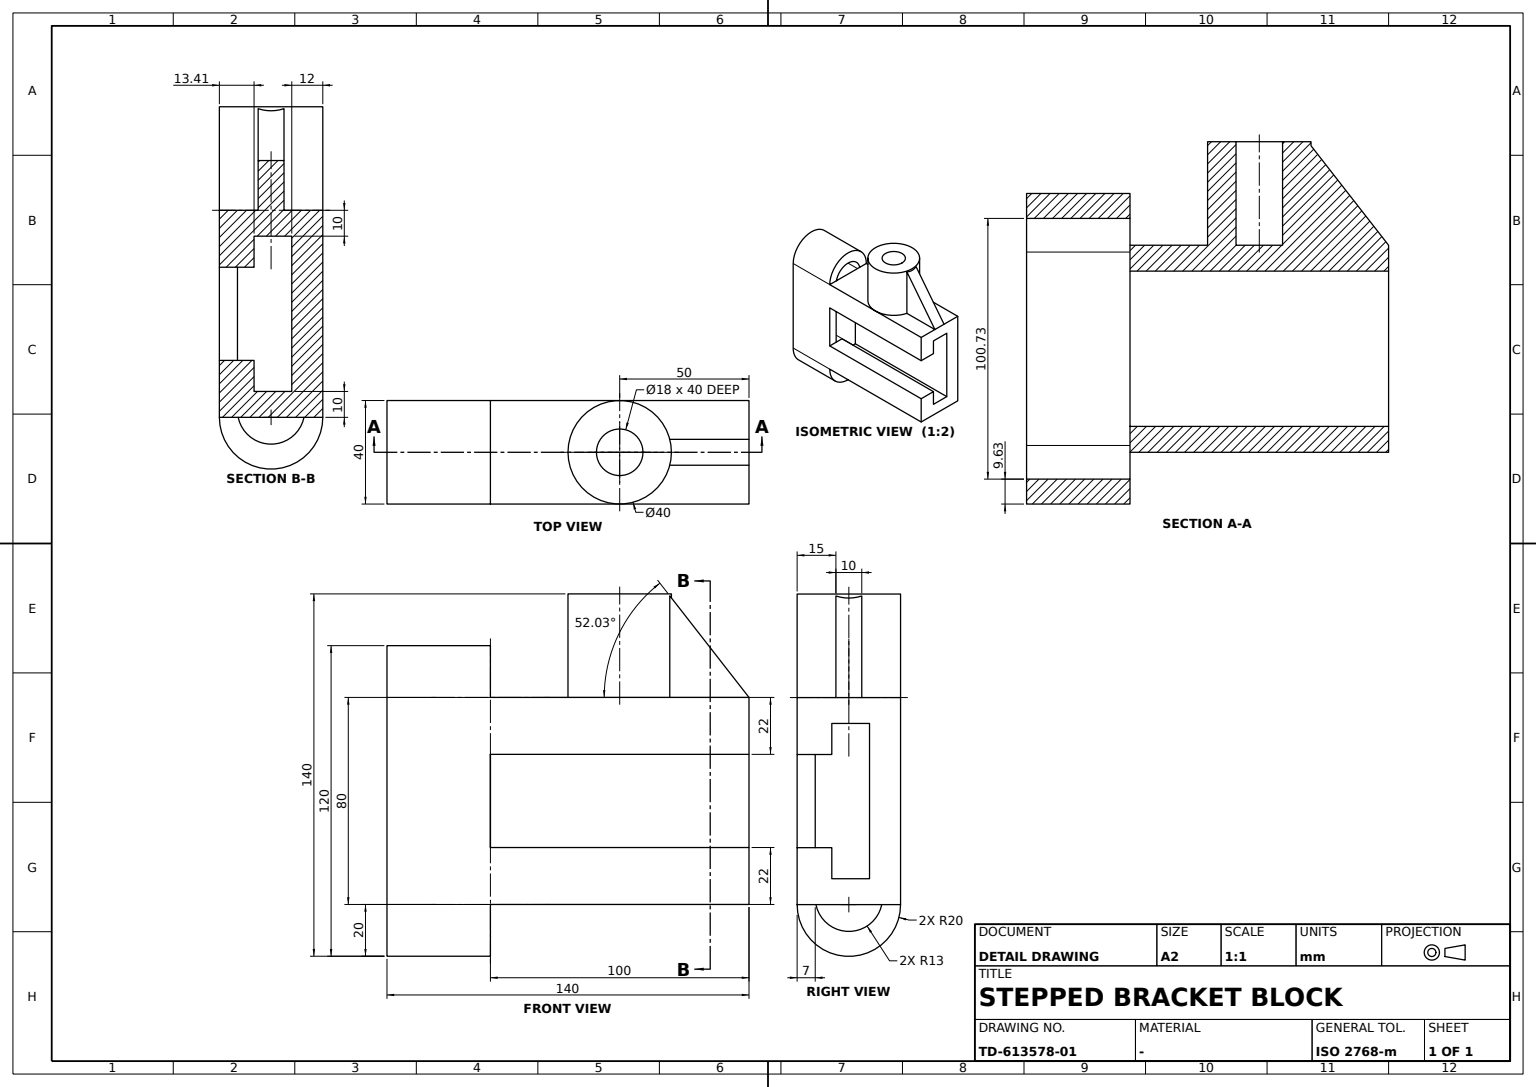
ISO-10303-21;
HEADER;
FILE_DESCRIPTION((''),'2;1');
FILE_NAME('','',(''),(''),'','','');
FILE_SCHEMA(('AUTOMOTIVE_DESIGN'));
ENDSEC;
DATA;
#1=APPLICATION_CONTEXT('');
#2=PRODUCT_CONTEXT('',#1,'mechanical');
#3=PRODUCT('','','',(#2));
#4=PRODUCT_DEFINITION_FORMATION('','',#3);
#5=PRODUCT_DEFINITION_CONTEXT('',#1,'design');
#6=PRODUCT_DEFINITION('','',#4,#5);
#7=PRODUCT_DEFINITION_SHAPE('','',#6);
#8=(LENGTH_UNIT()NAMED_UNIT(*)SI_UNIT(.MILLI.,.METRE.));
#9=(NAMED_UNIT(*)PLANE_ANGLE_UNIT()SI_UNIT($,.RADIAN.));
#10=(NAMED_UNIT(*)SI_UNIT($,.STERADIAN.)SOLID_ANGLE_UNIT());
#11=UNCERTAINTY_MEASURE_WITH_UNIT(LENGTH_MEASURE(0.005),#8,'distance_accuracy_value','');
#12=(GEOMETRIC_REPRESENTATION_CONTEXT(3)GLOBAL_UNCERTAINTY_ASSIGNED_CONTEXT((#11))GLOBAL_UNIT_ASSIGNED_CONTEXT((#8,#9,#10))REPRESENTATION_CONTEXT('',''));
#13=CARTESIAN_POINT('',(-41.,0.,40.));
#14=VERTEX_POINT('',#13);
#15=CARTESIAN_POINT('',(-50.,0.,40.));
#16=DIRECTION('',(0.,0.,1.));
#17=DIRECTION('',(1.,0.,0.));
#18=AXIS2_PLACEMENT_3D('',#15,#16,#17);
#19=CIRCLE('',#18,9.);
#20=EDGE_CURVE('',#14,#14,#19,.T.);
#21=ORIENTED_EDGE('',*,*,#20,.F.);
#22=EDGE_LOOP('',(#21));
#23=FACE_BOUND('',#22,.T.);
#24=CARTESIAN_POINT('',(-41.,0.,80.));
#25=VERTEX_POINT('',#24);
#26=CARTESIAN_POINT('',(-50.,0.,80.));
#27=AXIS2_PLACEMENT_3D('',#26,#16,#17);
#28=CIRCLE('',#27,9.);
#29=EDGE_CURVE('',#25,#25,#28,.T.);
#30=ORIENTED_EDGE('',*,*,#29,.T.);
#31=EDGE_LOOP('',(#30));
#32=FACE_BOUND('',#31,.T.);
#33=CARTESIAN_POINT('',(-50.,0.,60.));
#34=AXIS2_PLACEMENT_3D('',#33,#16,#17);
#35=CYLINDRICAL_SURFACE('',#34,9.);
#36=ADVANCED_FACE('',(#23,#32),#35,.F.);
#37=CARTESIAN_POINT('',(-100.,12.730269,40.));
#38=VERTEX_POINT('',#37);
#39=CARTESIAN_POINT('',(-100.,20.,40.));
#40=VERTEX_POINT('',#39);
#41=CARTESIAN_POINT('',(-100.,-20.,40.));
#42=DIRECTION('',(0.,1.,0.));
#43=VECTOR('',#42,1000.);
#44=LINE('',#41,#43);
#45=EDGE_CURVE('',#38,#40,#44,.T.);
#46=ORIENTED_EDGE('',*,*,#45,.T.);
#47=VERTEX_POINT('',#41);
#48=CARTESIAN_POINT('',(-100.,0.,40.));
#49=DIRECTION('',(0.,0.,-1.));
#50=AXIS2_PLACEMENT_3D('',#48,#17,#49);
#51=CIRCLE('',#50,20.);
#52=EDGE_CURVE('',#40,#47,#51,.T.);
#53=ORIENTED_EDGE('',*,*,#52,.T.);
#54=CARTESIAN_POINT('',(-100.,-12.730269,40.));
#55=VERTEX_POINT('',#54);
#56=EDGE_CURVE('',#47,#55,#44,.T.);
#57=ORIENTED_EDGE('',*,*,#56,.T.);
#58=CARTESIAN_POINT('',(-100.,0.,37.365564));
#59=AXIS2_PLACEMENT_3D('',#58,#17,#49);
#60=CIRCLE('',#59,13.);
#61=EDGE_CURVE('',#55,#38,#60,.F.);
#62=ORIENTED_EDGE('',*,*,#61,.T.);
#63=EDGE_LOOP('',(#46,#53,#57,#62));
#64=FACE_BOUND('',#63,.T.);
#65=CARTESIAN_POINT('',(-100.,0.,0.));
#66=AXIS2_PLACEMENT_3D('',#65,#17,#42);
#67=PLANE('',#66);
#68=ADVANCED_FACE('',(#64),#67,.T.);
#69=CARTESIAN_POINT('',(-100.,13.,-37.365564));
#70=VERTEX_POINT('',#69);
#71=CARTESIAN_POINT('',(-100.,12.730269,-40.));
#72=VERTEX_POINT('',#71);
#73=CARTESIAN_POINT('',(-100.,0.,-37.365564));
#74=AXIS2_PLACEMENT_3D('',#73,#17,#49);
#75=CIRCLE('',#74,13.);
#76=EDGE_CURVE('',#70,#72,#75,.F.);
#77=ORIENTED_EDGE('',*,*,#76,.F.);
#78=CARTESIAN_POINT('',(-140.,13.,-37.365564));
#79=VERTEX_POINT('',#78);
#80=CARTESIAN_POINT('',(-120.,13.,-37.365564));
#81=DIRECTION('',(-1.,0.,0.));
#82=VECTOR('',#81,1000.);
#83=LINE('',#80,#82);
#84=EDGE_CURVE('',#79,#70,#83,.F.);
#85=ORIENTED_EDGE('',*,*,#84,.F.);
#86=CARTESIAN_POINT('',(-140.,-13.,-37.365564));
#87=VERTEX_POINT('',#86);
#88=CARTESIAN_POINT('',(-140.,0.,-37.365564));
#89=AXIS2_PLACEMENT_3D('',#88,#81,#16);
#90=CIRCLE('',#89,13.);
#91=EDGE_CURVE('',#79,#87,#90,.T.);
#92=ORIENTED_EDGE('',*,*,#91,.T.);
#93=CARTESIAN_POINT('',(-100.,-13.,-37.365564));
#94=VERTEX_POINT('',#93);
#95=CARTESIAN_POINT('',(-120.,-13.,-37.365564));
#96=LINE('',#95,#82);
#97=EDGE_CURVE('',#87,#94,#96,.F.);
#98=ORIENTED_EDGE('',*,*,#97,.T.);
#99=CARTESIAN_POINT('',(-100.,-12.730269,-40.));
#100=VERTEX_POINT('',#99);
#101=EDGE_CURVE('',#100,#94,#75,.F.);
#102=ORIENTED_EDGE('',*,*,#101,.F.);
#103=EDGE_CURVE('',#72,#100,#75,.F.);
#104=ORIENTED_EDGE('',*,*,#103,.F.);
#105=EDGE_LOOP('',(#77,#85,#92,#98,#102,#104));
#106=FACE_BOUND('',#105,.T.);
#107=CARTESIAN_POINT('',(-120.,0.,-37.365564));
#108=DIRECTION('',(0.,-1.,0.));
#109=AXIS2_PLACEMENT_3D('',#107,#81,#108);
#110=CYLINDRICAL_SURFACE('',#109,13.);
#111=ADVANCED_FACE('',(#106),#110,.F.);
#112=CARTESIAN_POINT('',(-100.,-6.587677,30.));
#113=VERTEX_POINT('',#112);
#114=CARTESIAN_POINT('',(-100.,-6.587677,18.));
#115=VERTEX_POINT('',#114);
#116=VECTOR('',#49,1000.);
#117=LINE('',#112,#116);
#118=EDGE_CURVE('',#113,#115,#117,.T.);
#119=ORIENTED_EDGE('',*,*,#118,.F.);
#120=CARTESIAN_POINT('',(0.,-6.587677,30.));
#121=VERTEX_POINT('',#120);
#122=LINE('',#120,#82);
#123=EDGE_CURVE('',#121,#113,#122,.T.);
#124=ORIENTED_EDGE('',*,*,#123,.F.);
#125=CARTESIAN_POINT('',(0.,-6.587677,18.));
#126=VERTEX_POINT('',#125);
#127=LINE('',#120,#116);
#128=EDGE_CURVE('',#121,#126,#127,.T.);
#129=ORIENTED_EDGE('',*,*,#128,.T.);
#130=LINE('',#125,#82);
#131=EDGE_CURVE('',#126,#115,#130,.T.);
#132=ORIENTED_EDGE('',*,*,#131,.T.);
#133=EDGE_LOOP('',(#119,#124,#129,#132));
#134=FACE_BOUND('',#133,.T.);
#135=AXIS2_PLACEMENT_3D('',#120,#42,#49);
#136=PLANE('',#135);
#137=ADVANCED_FACE('',(#134),#136,.T.);
#138=CARTESIAN_POINT('',(-30.635083,-5.,40.));
#139=VERTEX_POINT('',#138);
#140=CARTESIAN_POINT('',(-30.635083,-5.,79.256793));
#141=VERTEX_POINT('',#140);
#142=VECTOR('',#16,1000.);
#143=LINE('',#138,#142);
#144=EDGE_CURVE('',#139,#141,#143,.T.);
#145=ORIENTED_EDGE('',*,*,#144,.T.);
#146=CARTESIAN_POINT('',(-30.635083,5.,79.256793));
#147=VERTEX_POINT('',#146);
#148=CARTESIAN_POINT('',(-50.,0.,104.071627));
#149=DIRECTION('',(0.788358294,0.,0.615216385));
#150=DIRECTION('',(-0.615216385,0.,0.788358294));
#151=AXIS2_PLACEMENT_3D('',#148,#149,#150);
#152=ELLIPSE('',#151,32.508887,20.);
#153=EDGE_CURVE('',#141,#147,#152,.T.);
#154=ORIENTED_EDGE('',*,*,#153,.T.);
#155=CARTESIAN_POINT('',(-30.635083,5.,40.));
#156=VERTEX_POINT('',#155);
#157=LINE('',#155,#142);
#158=EDGE_CURVE('',#156,#147,#157,.T.);
#159=ORIENTED_EDGE('',*,*,#158,.F.);
#160=CARTESIAN_POINT('',(-50.,20.,40.));
#161=VERTEX_POINT('',#160);
#162=CIRCLE('',#18,20.);
#163=EDGE_CURVE('',#156,#161,#162,.T.);
#164=ORIENTED_EDGE('',*,*,#163,.T.);
#165=CARTESIAN_POINT('',(-50.,-20.,40.));
#166=VERTEX_POINT('',#165);
#167=EDGE_CURVE('',#161,#166,#162,.T.);
#168=ORIENTED_EDGE('',*,*,#167,.T.);
#169=EDGE_CURVE('',#166,#139,#162,.T.);
#170=ORIENTED_EDGE('',*,*,#169,.T.);
#171=EDGE_LOOP('',(#145,#154,#159,#164,#168,#170));
#172=FACE_BOUND('',#171,.T.);
#173=CARTESIAN_POINT('',(-30.,0.,80.));
#174=VERTEX_POINT('',#173);
#175=CIRCLE('',#27,20.);
#176=EDGE_CURVE('',#174,#174,#175,.T.);
#177=ORIENTED_EDGE('',*,*,#176,.F.);
#178=EDGE_LOOP('',(#177));
#179=FACE_BOUND('',#178,.T.);
#180=CYLINDRICAL_SURFACE('',#34,20.);
#181=ADVANCED_FACE('',(#172,#179),#180,.T.);
#182=CARTESIAN_POINT('',(-140.,-13.,37.365564));
#183=VERTEX_POINT('',#182);
#184=CARTESIAN_POINT('',(-140.,13.,37.365564));
#185=VERTEX_POINT('',#184);
#186=CARTESIAN_POINT('',(-140.,0.,37.365564));
#187=AXIS2_PLACEMENT_3D('',#186,#81,#16);
#188=CIRCLE('',#187,13.);
#189=EDGE_CURVE('',#183,#185,#188,.T.);
#190=ORIENTED_EDGE('',*,*,#189,.T.);
#191=CARTESIAN_POINT('',(-100.,13.,37.365564));
#192=VERTEX_POINT('',#191);
#193=CARTESIAN_POINT('',(-120.,13.,37.365564));
#194=LINE('',#193,#82);
#195=EDGE_CURVE('',#185,#192,#194,.F.);
#196=ORIENTED_EDGE('',*,*,#195,.T.);
#197=EDGE_CURVE('',#38,#192,#60,.F.);
#198=ORIENTED_EDGE('',*,*,#197,.F.);
#199=ORIENTED_EDGE('',*,*,#61,.F.);
#200=CARTESIAN_POINT('',(-100.,-13.,37.365564));
#201=VERTEX_POINT('',#200);
#202=EDGE_CURVE('',#201,#55,#60,.F.);
#203=ORIENTED_EDGE('',*,*,#202,.F.);
#204=CARTESIAN_POINT('',(-120.,-13.,37.365564));
#205=LINE('',#204,#82);
#206=EDGE_CURVE('',#183,#201,#205,.F.);
#207=ORIENTED_EDGE('',*,*,#206,.F.);
#208=EDGE_LOOP('',(#190,#196,#198,#199,#203,#207));
#209=FACE_BOUND('',#208,.T.);
#210=CARTESIAN_POINT('',(-120.,0.,37.365564));
#211=AXIS2_PLACEMENT_3D('',#210,#81,#108);
#212=CYLINDRICAL_SURFACE('',#211,13.);
#213=ADVANCED_FACE('',(#209),#212,.F.);
#214=CARTESIAN_POINT('',(0.,5.,40.));
#215=VERTEX_POINT('',#214);
#216=CARTESIAN_POINT('',(19.400438,5.,15.139648));
#217=DIRECTION('',(0.615216385,0.,-0.788358294));
#218=VECTOR('',#217,1000.);
#219=LINE('',#216,#218);
#220=EDGE_CURVE('',#147,#215,#219,.T.);
#221=ORIENTED_EDGE('',*,*,#220,.T.);
#222=LINE('',#214,#82);
#223=EDGE_CURVE('',#215,#156,#222,.T.);
#224=ORIENTED_EDGE('',*,*,#223,.T.);
#225=ORIENTED_EDGE('',*,*,#158,.T.);
#226=EDGE_LOOP('',(#221,#224,#225));
#227=FACE_BOUND('',#226,.T.);
#228=CARTESIAN_POINT('',(0.,5.,0.));
#229=AXIS2_PLACEMENT_3D('',#228,#42,#81);
#230=PLANE('',#229);
#231=ADVANCED_FACE('',(#227),#230,.T.);
#232=CARTESIAN_POINT('',(-100.,-13.,-18.));
#233=VERTEX_POINT('',#232);
#234=CARTESIAN_POINT('',(-100.,-13.,0.));
#235=LINE('',#234,#142);
#236=EDGE_CURVE('',#94,#233,#235,.T.);
#237=ORIENTED_EDGE('',*,*,#236,.F.);
#238=ORIENTED_EDGE('',*,*,#97,.F.);
#239=LINE('',#86,#142);
#240=EDGE_CURVE('',#87,#183,#239,.T.);
#241=ORIENTED_EDGE('',*,*,#240,.T.);
#242=ORIENTED_EDGE('',*,*,#206,.T.);
#243=CARTESIAN_POINT('',(-100.,-13.,18.));
#244=VERTEX_POINT('',#243);
#245=EDGE_CURVE('',#244,#201,#235,.T.);
#246=ORIENTED_EDGE('',*,*,#245,.F.);
#247=EDGE_CURVE('',#233,#244,#235,.T.);
#248=ORIENTED_EDGE('',*,*,#247,.F.);
#249=EDGE_LOOP('',(#237,#238,#241,#242,#246,#248));
#250=FACE_BOUND('',#249,.T.);
#251=AXIS2_PLACEMENT_3D('',#86,#42,#16);
#252=PLANE('',#251);
#253=ADVANCED_FACE('',(#250),#252,.T.);
#254=ORIENTED_EDGE('',*,*,#202,.T.);
#255=EDGE_CURVE('',#55,#38,#44,.T.);
#256=ORIENTED_EDGE('',*,*,#255,.T.);
#257=ORIENTED_EDGE('',*,*,#197,.T.);
#258=CARTESIAN_POINT('',(-100.,13.,0.));
#259=LINE('',#258,#116);
#260=EDGE_CURVE('',#192,#70,#259,.T.);
#261=ORIENTED_EDGE('',*,*,#260,.T.);
#262=ORIENTED_EDGE('',*,*,#76,.T.);
#263=CARTESIAN_POINT('',(-100.,20.,-40.));
#264=VECTOR('',#108,1000.);
#265=LINE('',#263,#264);
#266=EDGE_CURVE('',#72,#100,#265,.T.);
#267=ORIENTED_EDGE('',*,*,#266,.T.);
#268=ORIENTED_EDGE('',*,*,#101,.T.);
#269=ORIENTED_EDGE('',*,*,#236,.T.);
#270=CARTESIAN_POINT('',(-100.,-6.587677,-18.));
#271=VERTEX_POINT('',#270);
#272=CARTESIAN_POINT('',(-100.,-20.,-18.));
#273=LINE('',#272,#43);
#274=EDGE_CURVE('',#233,#271,#273,.T.);
#275=ORIENTED_EDGE('',*,*,#274,.T.);
#276=CARTESIAN_POINT('',(-100.,-6.587677,-30.));
#277=VERTEX_POINT('',#276);
#278=EDGE_CURVE('',#271,#277,#117,.T.);
#279=ORIENTED_EDGE('',*,*,#278,.T.);
#280=CARTESIAN_POINT('',(-100.,8.,-30.));
#281=VERTEX_POINT('',#280);
#282=LINE('',#276,#43);
#283=EDGE_CURVE('',#277,#281,#282,.T.);
#284=ORIENTED_EDGE('',*,*,#283,.T.);
#285=CARTESIAN_POINT('',(-100.,8.,30.));
#286=VERTEX_POINT('',#285);
#287=LINE('',#280,#142);
#288=EDGE_CURVE('',#281,#286,#287,.T.);
#289=ORIENTED_EDGE('',*,*,#288,.T.);
#290=LINE('',#285,#264);
#291=EDGE_CURVE('',#286,#113,#290,.T.);
#292=ORIENTED_EDGE('',*,*,#291,.T.);
#293=ORIENTED_EDGE('',*,*,#118,.T.);
#294=LINE('',#114,#264);
#295=EDGE_CURVE('',#115,#244,#294,.T.);
#296=ORIENTED_EDGE('',*,*,#295,.T.);
#297=ORIENTED_EDGE('',*,*,#245,.T.);
#298=EDGE_LOOP('',(#254,#256,#257,#261,#262,#267,#268,#269,#275,#279,#284,#289,#292,#293,#296,#297));
#299=FACE_BOUND('',#298,.T.);
#300=ADVANCED_FACE('',(#299),#67,.F.);
#301=CARTESIAN_POINT('',(0.,8.,30.));
#302=VERTEX_POINT('',#301);
#303=LINE('',#301,#264);
#304=EDGE_CURVE('',#302,#121,#303,.T.);
#305=ORIENTED_EDGE('',*,*,#304,.T.);
#306=ORIENTED_EDGE('',*,*,#123,.T.);
#307=ORIENTED_EDGE('',*,*,#291,.F.);
#308=LINE('',#301,#82);
#309=EDGE_CURVE('',#302,#286,#308,.T.);
#310=ORIENTED_EDGE('',*,*,#309,.F.);
#311=EDGE_LOOP('',(#305,#306,#307,#310));
#312=FACE_BOUND('',#311,.T.);
#313=AXIS2_PLACEMENT_3D('',#301,#49,#108);
#314=PLANE('',#313);
#315=ADVANCED_FACE('',(#312),#314,.T.);
#316=LINE('',#184,#116);
#317=EDGE_CURVE('',#185,#79,#316,.T.);
#318=ORIENTED_EDGE('',*,*,#317,.F.);
#319=ORIENTED_EDGE('',*,*,#189,.F.);
#320=ORIENTED_EDGE('',*,*,#240,.F.);
#321=ORIENTED_EDGE('',*,*,#91,.F.);
#322=EDGE_LOOP('',(#318,#319,#320,#321));
#323=FACE_BOUND('',#322,.T.);
#324=CARTESIAN_POINT('',(-140.,-20.,-40.));
#325=VERTEX_POINT('',#324);
#326=CARTESIAN_POINT('',(-140.,-20.,40.));
#327=VERTEX_POINT('',#326);
#328=CARTESIAN_POINT('',(-140.,-20.,0.));
#329=LINE('',#328,#142);
#330=EDGE_CURVE('',#325,#327,#329,.T.);
#331=ORIENTED_EDGE('',*,*,#330,.T.);
#332=CARTESIAN_POINT('',(-140.,20.,40.));
#333=VERTEX_POINT('',#332);
#334=CARTESIAN_POINT('',(-140.,0.,40.));
#335=AXIS2_PLACEMENT_3D('',#334,#81,#16);
#336=CIRCLE('',#335,20.);
#337=EDGE_CURVE('',#333,#327,#336,.F.);
#338=ORIENTED_EDGE('',*,*,#337,.F.);
#339=CARTESIAN_POINT('',(-140.,20.,-40.));
#340=VERTEX_POINT('',#339);
#341=CARTESIAN_POINT('',(-140.,20.,0.));
#342=LINE('',#341,#116);
#343=EDGE_CURVE('',#333,#340,#342,.T.);
#344=ORIENTED_EDGE('',*,*,#343,.T.);
#345=CARTESIAN_POINT('',(-140.,0.,-40.));
#346=AXIS2_PLACEMENT_3D('',#345,#81,#16);
#347=CIRCLE('',#346,20.);
#348=EDGE_CURVE('',#325,#340,#347,.F.);
#349=ORIENTED_EDGE('',*,*,#348,.F.);
#350=EDGE_LOOP('',(#331,#338,#344,#349));
#351=FACE_BOUND('',#350,.T.);
#352=CARTESIAN_POINT('',(-140.,0.,0.));
#353=AXIS2_PLACEMENT_3D('',#352,#81,#108);
#354=PLANE('',#353);
#355=ADVANCED_FACE('',(#323,#351),#354,.T.);
#356=ORIENTED_EDGE('',*,*,#167,.F.);
#357=CARTESIAN_POINT('',(0.,20.,40.));
#358=LINE('',#357,#82);
#359=EDGE_CURVE('',#161,#40,#358,.T.);
#360=ORIENTED_EDGE('',*,*,#359,.T.);
#361=ORIENTED_EDGE('',*,*,#45,.F.);
#362=ORIENTED_EDGE('',*,*,#255,.F.);
#363=ORIENTED_EDGE('',*,*,#56,.F.);
#364=CARTESIAN_POINT('',(0.,-20.,40.));
#365=LINE('',#364,#82);
#366=EDGE_CURVE('',#166,#47,#365,.T.);
#367=ORIENTED_EDGE('',*,*,#366,.F.);
#368=EDGE_LOOP('',(#356,#360,#361,#362,#363,#367));
#369=FACE_BOUND('',#368,.T.);
#370=AXIS2_PLACEMENT_3D('',#364,#16,#42);
#371=PLANE('',#370);
#372=ADVANCED_FACE('',(#369),#371,.T.);
#373=ORIENTED_EDGE('',*,*,#52,.F.);
#374=CARTESIAN_POINT('',(-120.,20.,40.));
#375=VECTOR('',#17,1000.);
#376=LINE('',#374,#375);
#377=EDGE_CURVE('',#40,#333,#376,.F.);
#378=ORIENTED_EDGE('',*,*,#377,.T.);
#379=ORIENTED_EDGE('',*,*,#337,.T.);
#380=CARTESIAN_POINT('',(-120.,-20.,40.));
#381=LINE('',#380,#375);
#382=EDGE_CURVE('',#47,#327,#381,.F.);
#383=ORIENTED_EDGE('',*,*,#382,.F.);
#384=EDGE_LOOP('',(#373,#378,#379,#383));
#385=FACE_BOUND('',#384,.T.);
#386=CARTESIAN_POINT('',(-120.,0.,40.));
#387=AXIS2_PLACEMENT_3D('',#386,#17,#42);
#388=CYLINDRICAL_SURFACE('',#387,20.);
#389=ADVANCED_FACE('',(#385),#388,.T.);
#390=CARTESIAN_POINT('',(0.,-6.587677,-18.));
#391=VERTEX_POINT('',#390);
#392=LINE('',#390,#82);
#393=EDGE_CURVE('',#391,#271,#392,.T.);
#394=ORIENTED_EDGE('',*,*,#393,.T.);
#395=ORIENTED_EDGE('',*,*,#274,.F.);
#396=VERTEX_POINT('',#272);
#397=EDGE_CURVE('',#396,#233,#273,.T.);
#398=ORIENTED_EDGE('',*,*,#397,.F.);
#399=CARTESIAN_POINT('',(0.,-20.,-18.));
#400=VERTEX_POINT('',#399);
#401=LINE('',#399,#82);
#402=EDGE_CURVE('',#400,#396,#401,.T.);
#403=ORIENTED_EDGE('',*,*,#402,.F.);
#404=LINE('',#399,#43);
#405=EDGE_CURVE('',#400,#391,#404,.T.);
#406=ORIENTED_EDGE('',*,*,#405,.T.);
#407=EDGE_LOOP('',(#394,#395,#398,#403,#406));
#408=FACE_BOUND('',#407,.T.);
#409=AXIS2_PLACEMENT_3D('',#399,#16,#42);
#410=PLANE('',#409);
#411=ADVANCED_FACE('',(#408),#410,.T.);
#412=ORIENTED_EDGE('',*,*,#309,.T.);
#413=ORIENTED_EDGE('',*,*,#288,.F.);
#414=CARTESIAN_POINT('',(0.,8.,-30.));
#415=VERTEX_POINT('',#414);
#416=LINE('',#414,#82);
#417=EDGE_CURVE('',#415,#281,#416,.T.);
#418=ORIENTED_EDGE('',*,*,#417,.F.);
#419=LINE('',#414,#142);
#420=EDGE_CURVE('',#415,#302,#419,.T.);
#421=ORIENTED_EDGE('',*,*,#420,.T.);
#422=EDGE_LOOP('',(#412,#413,#418,#421));
#423=FACE_BOUND('',#422,.T.);
#424=AXIS2_PLACEMENT_3D('',#414,#108,#16);
#425=PLANE('',#424);
#426=ADVANCED_FACE('',(#423),#425,.T.);
#427=ORIENTED_EDGE('',*,*,#195,.F.);
#428=ORIENTED_EDGE('',*,*,#317,.T.);
#429=ORIENTED_EDGE('',*,*,#84,.T.);
#430=ORIENTED_EDGE('',*,*,#260,.F.);
#431=EDGE_LOOP('',(#427,#428,#429,#430));
#432=FACE_BOUND('',#431,.T.);
#433=AXIS2_PLACEMENT_3D('',#184,#108,#49);
#434=PLANE('',#433);
#435=ADVANCED_FACE('',(#432),#434,.T.);
#436=CARTESIAN_POINT('',(0.,-5.,40.));
#437=VERTEX_POINT('',#436);
#438=CARTESIAN_POINT('',(19.400438,-5.,15.139648));
#439=LINE('',#438,#218);
#440=EDGE_CURVE('',#141,#437,#439,.T.);
#441=ORIENTED_EDGE('',*,*,#440,.F.);
#442=ORIENTED_EDGE('',*,*,#144,.F.);
#443=LINE('',#436,#82);
#444=EDGE_CURVE('',#437,#139,#443,.T.);
#445=ORIENTED_EDGE('',*,*,#444,.F.);
#446=EDGE_LOOP('',(#441,#442,#445));
#447=FACE_BOUND('',#446,.T.);
#448=CARTESIAN_POINT('',(0.,-5.,0.));
#449=AXIS2_PLACEMENT_3D('',#448,#42,#81);
#450=PLANE('',#449);
#451=ADVANCED_FACE('',(#447),#450,.F.);
#452=CARTESIAN_POINT('',(0.,-20.,18.));
#453=VERTEX_POINT('',#452);
#454=VERTEX_POINT('',#364);
#455=LINE('',#452,#142);
#456=EDGE_CURVE('',#453,#454,#455,.T.);
#457=ORIENTED_EDGE('',*,*,#456,.F.);
#458=LINE('',#125,#264);
#459=EDGE_CURVE('',#126,#453,#458,.T.);
#460=ORIENTED_EDGE('',*,*,#459,.F.);
#461=ORIENTED_EDGE('',*,*,#128,.F.);
#462=ORIENTED_EDGE('',*,*,#304,.F.);
#463=ORIENTED_EDGE('',*,*,#420,.F.);
#464=CARTESIAN_POINT('',(0.,-6.587677,-30.));
#465=VERTEX_POINT('',#464);
#466=LINE('',#464,#43);
#467=EDGE_CURVE('',#465,#415,#466,.T.);
#468=ORIENTED_EDGE('',*,*,#467,.F.);
#469=EDGE_CURVE('',#391,#465,#127,.T.);
#470=ORIENTED_EDGE('',*,*,#469,.F.);
#471=ORIENTED_EDGE('',*,*,#405,.F.);
#472=CARTESIAN_POINT('',(0.,-20.,-40.));
#473=VERTEX_POINT('',#472);
#474=EDGE_CURVE('',#473,#400,#455,.T.);
#475=ORIENTED_EDGE('',*,*,#474,.F.);
#476=CARTESIAN_POINT('',(0.,20.,-40.));
#477=VERTEX_POINT('',#476);
#478=LINE('',#476,#264);
#479=EDGE_CURVE('',#477,#473,#478,.T.);
#480=ORIENTED_EDGE('',*,*,#479,.F.);
#481=VERTEX_POINT('',#357);
#482=LINE('',#357,#116);
#483=EDGE_CURVE('',#481,#477,#482,.T.);
#484=ORIENTED_EDGE('',*,*,#483,.F.);
#485=LINE('',#364,#43);
#486=EDGE_CURVE('',#215,#481,#485,.T.);
#487=ORIENTED_EDGE('',*,*,#486,.F.);
#488=CARTESIAN_POINT('',(0.,0.,40.));
#489=LINE('',#488,#43);
#490=EDGE_CURVE('',#437,#215,#489,.T.);
#491=ORIENTED_EDGE('',*,*,#490,.F.);
#492=EDGE_CURVE('',#454,#437,#485,.T.);
#493=ORIENTED_EDGE('',*,*,#492,.F.);
#494=EDGE_LOOP('',(#457,#460,#461,#462,#463,#468,#470,#471,#475,#480,#484,#487,#491,#493));
#495=FACE_BOUND('',#494,.T.);
#496=CARTESIAN_POINT('',(0.,0.,0.));
#497=AXIS2_PLACEMENT_3D('',#496,#17,#42);
#498=PLANE('',#497);
#499=ADVANCED_FACE('',(#495),#498,.T.);
#500=ORIENTED_EDGE('',*,*,#103,.T.);
#501=CARTESIAN_POINT('',(-100.,-20.,-40.));
#502=VERTEX_POINT('',#501);
#503=EDGE_CURVE('',#100,#502,#265,.T.);
#504=ORIENTED_EDGE('',*,*,#503,.T.);
#505=VERTEX_POINT('',#263);
#506=CARTESIAN_POINT('',(-100.,0.,-40.));
#507=AXIS2_PLACEMENT_3D('',#506,#17,#49);
#508=CIRCLE('',#507,20.);
#509=EDGE_CURVE('',#502,#505,#508,.T.);
#510=ORIENTED_EDGE('',*,*,#509,.T.);
#511=EDGE_CURVE('',#505,#72,#265,.T.);
#512=ORIENTED_EDGE('',*,*,#511,.T.);
#513=EDGE_LOOP('',(#500,#504,#510,#512));
#514=FACE_BOUND('',#513,.T.);
#515=ADVANCED_FACE('',(#514),#67,.T.);
#516=ORIENTED_EDGE('',*,*,#169,.F.);
#517=EDGE_CURVE('',#454,#166,#365,.T.);
#518=ORIENTED_EDGE('',*,*,#517,.F.);
#519=ORIENTED_EDGE('',*,*,#492,.T.);
#520=ORIENTED_EDGE('',*,*,#444,.T.);
#521=EDGE_LOOP('',(#516,#518,#519,#520));
#522=FACE_BOUND('',#521,.T.);
#523=ADVANCED_FACE('',(#522),#371,.T.);
#524=ORIENTED_EDGE('',*,*,#266,.F.);
#525=ORIENTED_EDGE('',*,*,#511,.F.);
#526=LINE('',#476,#82);
#527=EDGE_CURVE('',#477,#505,#526,.T.);
#528=ORIENTED_EDGE('',*,*,#527,.F.);
#529=ORIENTED_EDGE('',*,*,#479,.T.);
#530=LINE('',#472,#82);
#531=EDGE_CURVE('',#473,#502,#530,.T.);
#532=ORIENTED_EDGE('',*,*,#531,.T.);
#533=ORIENTED_EDGE('',*,*,#503,.F.);
#534=EDGE_LOOP('',(#524,#525,#528,#529,#532,#533));
#535=FACE_BOUND('',#534,.T.);
#536=AXIS2_PLACEMENT_3D('',#476,#49,#108);
#537=PLANE('',#536);
#538=ADVANCED_FACE('',(#535),#537,.T.);
#539=CARTESIAN_POINT('',(-100.,-20.,18.));
#540=VERTEX_POINT('',#539);
#541=EDGE_CURVE('',#244,#540,#294,.T.);
#542=ORIENTED_EDGE('',*,*,#541,.F.);
#543=ORIENTED_EDGE('',*,*,#295,.F.);
#544=ORIENTED_EDGE('',*,*,#131,.F.);
#545=ORIENTED_EDGE('',*,*,#459,.T.);
#546=LINE('',#452,#82);
#547=EDGE_CURVE('',#453,#540,#546,.T.);
#548=ORIENTED_EDGE('',*,*,#547,.T.);
#549=EDGE_LOOP('',(#542,#543,#544,#545,#548));
#550=FACE_BOUND('',#549,.T.);
#551=AXIS2_PLACEMENT_3D('',#125,#49,#108);
#552=PLANE('',#551);
#553=ADVANCED_FACE('',(#550),#552,.T.);
#554=ORIENTED_EDGE('',*,*,#486,.T.);
#555=EDGE_CURVE('',#481,#161,#358,.T.);
#556=ORIENTED_EDGE('',*,*,#555,.T.);
#557=ORIENTED_EDGE('',*,*,#163,.F.);
#558=ORIENTED_EDGE('',*,*,#223,.F.);
#559=EDGE_LOOP('',(#554,#556,#557,#558));
#560=FACE_BOUND('',#559,.T.);
#561=ADVANCED_FACE('',(#560),#371,.T.);
#562=ORIENTED_EDGE('',*,*,#220,.F.);
#563=ORIENTED_EDGE('',*,*,#153,.F.);
#564=ORIENTED_EDGE('',*,*,#440,.T.);
#565=ORIENTED_EDGE('',*,*,#490,.T.);
#566=EDGE_LOOP('',(#562,#563,#564,#565));
#567=FACE_BOUND('',#566,.T.);
#568=CARTESIAN_POINT('',(-31.215065,0.,80.));
#569=AXIS2_PLACEMENT_3D('',#568,#149,#217);
#570=PLANE('',#569);
#571=ADVANCED_FACE('',(#567),#570,.T.);
#572=ORIENTED_EDGE('',*,*,#29,.F.);
#573=EDGE_LOOP('',(#572));
#574=FACE_BOUND('',#573,.T.);
#575=ORIENTED_EDGE('',*,*,#176,.T.);
#576=EDGE_LOOP('',(#575));
#577=FACE_BOUND('',#576,.T.);
#578=CARTESIAN_POINT('',(0.,0.,80.));
#579=AXIS2_PLACEMENT_3D('',#578,#16,#17);
#580=PLANE('',#579);
#581=ADVANCED_FACE('',(#574,#577),#580,.T.);
#582=ORIENTED_EDGE('',*,*,#541,.T.);
#583=LINE('',#539,#142);
#584=EDGE_CURVE('',#396,#540,#583,.T.);
#585=ORIENTED_EDGE('',*,*,#584,.F.);
#586=ORIENTED_EDGE('',*,*,#397,.T.);
#587=ORIENTED_EDGE('',*,*,#247,.T.);
#588=EDGE_LOOP('',(#582,#585,#586,#587));
#589=FACE_BOUND('',#588,.T.);
#590=ADVANCED_FACE('',(#589),#67,.T.);
#591=LINE('',#464,#82);
#592=EDGE_CURVE('',#465,#277,#591,.T.);
#593=ORIENTED_EDGE('',*,*,#592,.F.);
#594=ORIENTED_EDGE('',*,*,#467,.T.);
#595=ORIENTED_EDGE('',*,*,#417,.T.);
#596=ORIENTED_EDGE('',*,*,#283,.F.);
#597=EDGE_LOOP('',(#593,#594,#595,#596));
#598=FACE_BOUND('',#597,.T.);
#599=AXIS2_PLACEMENT_3D('',#464,#16,#42);
#600=PLANE('',#599);
#601=ADVANCED_FACE('',(#598),#600,.T.);
#602=CARTESIAN_POINT('',(-120.,-20.,-40.));
#603=LINE('',#602,#375);
#604=EDGE_CURVE('',#502,#325,#603,.F.);
#605=ORIENTED_EDGE('',*,*,#604,.T.);
#606=ORIENTED_EDGE('',*,*,#348,.T.);
#607=CARTESIAN_POINT('',(-120.,20.,-40.));
#608=LINE('',#607,#375);
#609=EDGE_CURVE('',#505,#340,#608,.F.);
#610=ORIENTED_EDGE('',*,*,#609,.F.);
#611=ORIENTED_EDGE('',*,*,#509,.F.);
#612=EDGE_LOOP('',(#605,#606,#610,#611));
#613=FACE_BOUND('',#612,.T.);
#614=CARTESIAN_POINT('',(-120.,0.,-40.));
#615=AXIS2_PLACEMENT_3D('',#614,#17,#42);
#616=CYLINDRICAL_SURFACE('',#615,20.);
#617=ADVANCED_FACE('',(#613),#616,.T.);
#618=ORIENTED_EDGE('',*,*,#20,.T.);
#619=EDGE_LOOP('',(#618));
#620=FACE_BOUND('',#619,.T.);
#621=ADVANCED_FACE('',(#620),#371,.T.);
#622=ORIENTED_EDGE('',*,*,#359,.F.);
#623=ORIENTED_EDGE('',*,*,#555,.F.);
#624=ORIENTED_EDGE('',*,*,#483,.T.);
#625=ORIENTED_EDGE('',*,*,#527,.T.);
#626=ORIENTED_EDGE('',*,*,#609,.T.);
#627=ORIENTED_EDGE('',*,*,#343,.F.);
#628=ORIENTED_EDGE('',*,*,#377,.F.);
#629=EDGE_LOOP('',(#622,#623,#624,#625,#626,#627,#628));
#630=FACE_BOUND('',#629,.T.);
#631=AXIS2_PLACEMENT_3D('',#357,#42,#49);
#632=PLANE('',#631);
#633=ADVANCED_FACE('',(#630),#632,.T.);
#634=ORIENTED_EDGE('',*,*,#456,.T.);
#635=ORIENTED_EDGE('',*,*,#517,.T.);
#636=ORIENTED_EDGE('',*,*,#366,.T.);
#637=ORIENTED_EDGE('',*,*,#382,.T.);
#638=ORIENTED_EDGE('',*,*,#330,.F.);
#639=ORIENTED_EDGE('',*,*,#604,.F.);
#640=ORIENTED_EDGE('',*,*,#531,.F.);
#641=ORIENTED_EDGE('',*,*,#474,.T.);
#642=ORIENTED_EDGE('',*,*,#402,.T.);
#643=ORIENTED_EDGE('',*,*,#584,.T.);
#644=ORIENTED_EDGE('',*,*,#547,.F.);
#645=EDGE_LOOP('',(#634,#635,#636,#637,#638,#639,#640,#641,#642,#643,#644));
#646=FACE_BOUND('',#645,.T.);
#647=AXIS2_PLACEMENT_3D('',#452,#108,#16);
#648=PLANE('',#647);
#649=ADVANCED_FACE('',(#646),#648,.T.);
#650=ORIENTED_EDGE('',*,*,#278,.F.);
#651=ORIENTED_EDGE('',*,*,#393,.F.);
#652=ORIENTED_EDGE('',*,*,#469,.T.);
#653=ORIENTED_EDGE('',*,*,#592,.T.);
#654=EDGE_LOOP('',(#650,#651,#652,#653));
#655=FACE_BOUND('',#654,.T.);
#656=ADVANCED_FACE('',(#655),#136,.T.);
#657=CLOSED_SHELL('',(#36,#68,#111,#137,#181,#213,#231,#253,#300,#315,#355,#372,#389,#411,#426,#435,#451,#499,#515,#523,#538,#553,#561,#571,#581,#590,#601,#617,#621,#633,#649,#656));
#658=MANIFOLD_SOLID_BREP('',#657);
#659=ADVANCED_BREP_SHAPE_REPRESENTATION('',(#658),#12);
#660=SHAPE_DEFINITION_REPRESENTATION(#7,#659);
ENDSEC;
END-ISO-10303-21;
